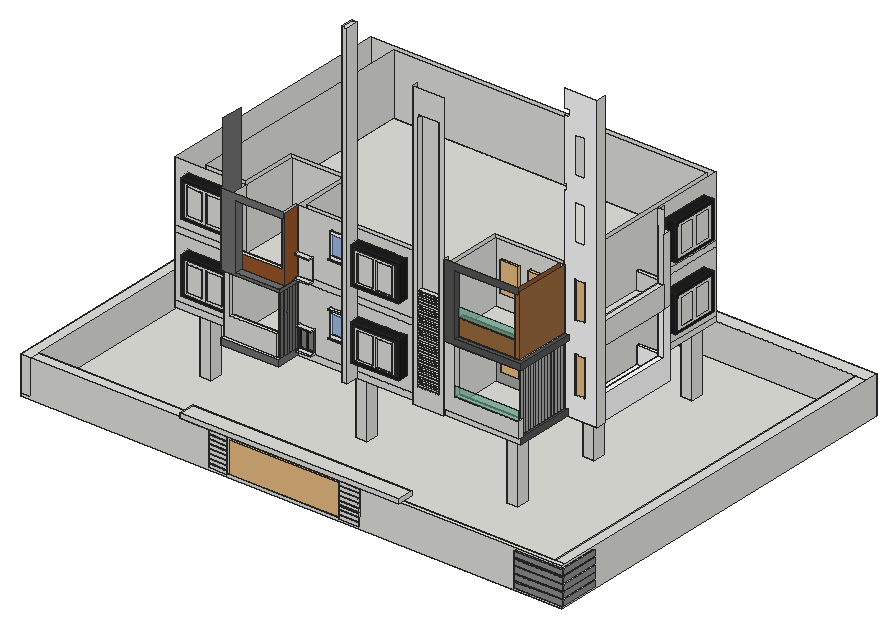
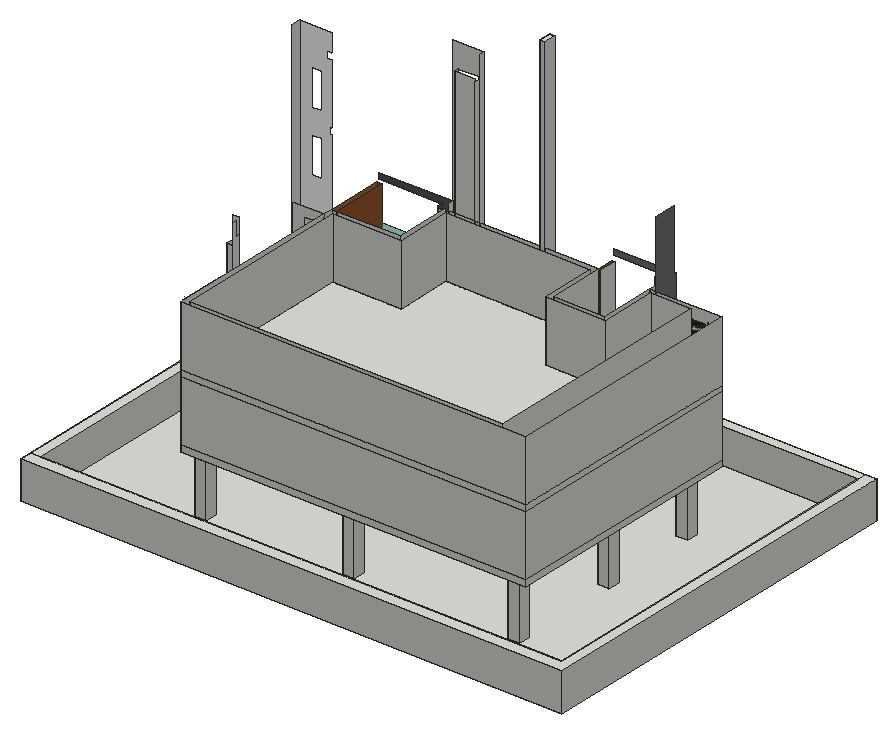
# SketchUp Ruby script. Lengths in inches.
U = 1.inch
M = Sketchup.active_model
def pt(a) = Geom::Point3d.new(a.map { |v| v * U })
def face(e, loops, mat)
  f = e.add_face(loops[0].map { |a| pt(a) })
  loops[1..].each { |l| e.add_face(l.map { |a| pt(a) }).erase! }
  f.material = f.back_material = mat if mat
  f
end
# faces: each face lists its corners as indices into pts; further lists are holes
def faces(e, pts, list, mat = nil) = list.each { |f| face(e, (f[0].is_a?(Array) ? f : [f]).map { |l| l.map { |i| pts[i] } }, mat) }
# xy, xz, yz: faces in a plane at the given z, y or x. An outline is a flat list of corners, or four numbers for a rectangle; further outlines are holes
def ring(l) = l.size == 4 ? [[l[0], l[1]], [l[2], l[1]], [l[2], l[3]], [l[0], l[3]]] : l.each_slice(2).to_a
def flat(e, list, mat, &to3) = list.each { |f| face(e, (f[0].is_a?(Array) ? f : [f]).map { |l| ring(l).map { |u, v| to3.(u, v) } }, mat) }
def xy(e, z, list, mat = nil) = flat(e, list, mat) { |x, y| [x, y, z] }
def xz(e, y, list, mat = nil) = flat(e, list, mat) { |x, z| [x, y, z] }
def yz(e, x, list, mat = nil) = flat(e, list, mat) { |y, z| [x, y, z] }
def lines(e, pts, list) = list.each { |a, b| e.add_line(pt(pts[a]), pt(pts[b])) }
# prism: a flat outline (further loops are holes) pulled along v
def prism(e, loops, v, mat = nil)
  f = face(e, loops, mat); d = Geom::Vector3d.new(v.map { |x| x * U })
  f.pushpull(f.normal.samedirection?(d) ? d.length : -d.length)
end
def box(e, o, s, mat = nil) = prism(e, [[o, [o[0] + s[0], o[1], o[2]], [o[0] + s[0], o[1] + s[1], o[2]], [o[0], o[1] + s[1], o[2]]]], [0, 0, s[2]], mat)
def at(x, y, z, deg = 0) = Geom::Transformation.translation(pt([x, y, z])) * Geom::Transformation.rotation(ORIGIN, Z_AXIS, deg.degrees)
def axes(o, x, y, z) = Geom::Transformation.new([*x, 0, *y, 0, *z, 0, *pt(o).to_a, 1])
def part(name) = M.definitions.add(name)
# library, detail: a bought-in or finely detailed component or shape, given as its bounding box
def library(name, o, s) = part(name).tap { |d| box(d.entities, o, s) }
def detail(e, o, s) = box(e.add_group.entities, o, s)
def put(e, d, t, mat = nil) = e.add_instance(d, t).tap { |i| i.material = mat if mat }
def group(e, t, mat = nil) = e.add_group.tap { |g| g.transformation = t; g.material = mat if mat }.entities
root = M.entities
M.materials.add("Glass_Tinted_Gray").color = [0, 0, 0]
M.materials["Glass_Tinted_Gray"].alpha = 0.125
M.materials.add("MaterialE").color = [182, 131, 172]
M.materials["MaterialE"].alpha = 0.66
M.materials.add("MaterialF").color = [114, 188, 161]
M.materials["MaterialF"].alpha = 0.66
M.materials.add("[0135_DarkGray]").color = [81, 81, 81]
M.materials.add("[Color M00]").color = [255, 255, 255]
M.materials.add("[Color M03]").color = [170, 170, 170]
M.materials.add("[Color M04]").color = [142, 142, 142]
M.materials.add("[Color M05]").color = [114, 114, 114]
M.materials.add("[Color M06]").color = [86, 86, 86]
M.materials.add("[Color M08]").color = [30, 30, 30]
M.materials.add("[Color_000]").color = [255, 255, 255]
M.materials.add("[Mirror 02]1").color = [229, 229, 229]
M.materials.add("[Terrazzo Light Blue]").color = [196, 214, 227]
M.materials.add("[Translucent Glass Blue]").color = [100, 149, 237]
M.materials["[Translucent Glass Blue]"].alpha = 0.5
M.materials.add("[Wood Cherry Original]").color = [152, 86, 42]
M.materials.add("[Wood Floor]").color = [155, 105, 61]
c1 = part("Group\#83")
box(c1.entities,[-12.25,0,-120],[22.4375,23.375,120])
c2 = library("Slatted gate assembly",[-0.09,68.76,-0.1],[160,5.32,60.06])
c3 = part("Group\#96")
box(c3.entities,[0,-1.1875,0],[36.6875,1.1875,6.49])
c4 = part("Group\#3")
box(c4.entities,[3,0,0],[2.8125,4.1875,120.875])
c5 = part("Group\#76")
box(c5.entities,[0,0,0],[4.8125,4.8125,120],"[Color M05]")
c6 = library("Single door",[0,0,0],[7.5,39.86,83.92])
c7 = part("Group\#75")
box(c7.entities,[0,-10.375,0],[28.375,10.375,2.5])
c8 = part("PENTEK_RP Fineline 50S_Sliding_DoorCase_E1")
box(c8.entities,[0,0,0],[1.51,3.66,99.27],"[0135_DarkGray]")
c9 = part("PENTEK_RP Fineline 50S_SlidingDooe_Case_E2")
box(c9.entities,[0,0,0],[96.25,3.66,1.51],"[0135_DarkGray]")
c10 = part("pentek_RP Fineline 50S_SlidingDoor_Case")
put(c10.entities,c8,at(97.76,0,0))
put(c10.entities,c9,at(1.51,0,0))
put(c10.entities,c8,at(0,0,0))
put(c10.entities,c9,at(1.51,0,97.76))
c11 = part("PENTEK_RP Fineline 50S_SlidingDoor_GlazingBead_2")
box(c11.entities,[0,0,0],[0.56,0.59,94.39],"[0135_DarkGray]")
c12 = part("PENTEK_RP Fineline 50S_SlidingDoor_Glass")
box(c12.entities,[0,0,0],[46.58,0.16,94.39],"Glass_Tinted_Gray")
c13 = part("PENTEK_RP Fineline 50S_SlidingDoor_GlazingBead")
box(c13.entities,[0,0,0],[45.47,0.59,0.56],"[0135_DarkGray]")
c14 = part("PENTEK_RP Fineline 50S_SlidingDoor_Leaf_E1")
xy(c14.entities,0,[[0,0,0.93,1.97],[0.93,1.57,1.49,1.97]],"[0135_DarkGray]")
xy(c14.entities,96.25,[[0,0,0.93,0,0.93,1.57,1.49,1.57,1.49,1.97,0,1.97]],"[0135_DarkGray]")
xz(c14.entities,0,[[0,0,0.93,96.25]],"[0135_DarkGray]")
xz(c14.entities,1.57,[[0.93,0,1.49,95.32],[0.93,95.32,1.49,96.25]],"[0135_DarkGray]")
xz(c14.entities,1.97,[[0,0,1.49,96.25]],"[0135_DarkGray]")
yz(c14.entities,0,[[0,0,1.97,96.25]],"[0135_DarkGray]")
yz(c14.entities,0.93,[[0,0,1.57,0.93],[0,0.93,1.57,95.32],[0,95.32,1.57,96.25]],"[0135_DarkGray]")
yz(c14.entities,1.49,[[1.57,0,1.97,95.32],[1.57,95.32,1.97,96.25]],"[0135_DarkGray]")
c15 = part("PENTEK_RP Fineline 50S_SlidingDoor_Leaf_E2")
xy(c15.entities,0,[[0,0,0,1.57,0.56,1.57,0.56,1.97,46.02,1.97,46.02,1.57,46.58,1.57,46.58,0]],"[0135_DarkGray]")
xy(c15.entities,0.93,[[0,0,46.58,1.57]],"[0135_DarkGray]")
xy(c15.entities,1.49,[[0.56,1.57,46.02,1.97]],"[0135_DarkGray]")
xz(c15.entities,0,[[0,0,46.58,0.93]],"[0135_DarkGray]")
xz(c15.entities,1.57,[[0,0,0.56,0.93],[46.02,0,46.58,0.93],[0.56,0.93,46.02,1.49]],"[0135_DarkGray]")
xz(c15.entities,1.97,[[0.56,0,46.02,1.49]],"[0135_DarkGray]")
yz(c15.entities,0,[[0,0,1.57,0.93]],"[0135_DarkGray]")
yz(c15.entities,0.56,[[1.57,0,1.97,0.93],[1.57,0.93,1.97,1.49]],"[0135_DarkGray]")
yz(c15.entities,46.02,[[1.57,0,1.97,0.93],[1.57,0.93,1.97,1.49]],"[0135_DarkGray]")
yz(c15.entities,46.58,[[0,0,1.57,0.93]],"[0135_DarkGray]")
c16 = part("PENTEK_RP Fineline S_SlidingDoor_Leaf1")
put(c16.entities,c11,at(0.93,0,0.93))
put(c16.entities,c11,at(46.96,0,0.93))
put(c16.entities,c12,at(1.49,1.42,0.93))
put(c16.entities,c13,at(1.49,0,0.93))
put(c16.entities,c12,at(1.49,0.59,0.93),"[Terrazzo Light Blue]")
put(c16.entities,c14,at(0,0,0))
put(c16.entities,c14,axes([48.44,0,0],[-1,0,0],[0,1,0],[0,0,1]))
put(c16.entities,c15,axes([0.93,0,96.25],[1,0,0],[0,1,0],[0,0,-1]))
put(c16.entities,c15,at(0.93,0,0))
put(c16.entities,c13,at(1.49,0,94.77))
c17 = part("PENTEK_RP Fineline 50S_SlidingDoor_Leaf2")
put(c17.entities,c12,at(1.49,1.42,0.93))
put(c17.entities,c13,at(1.49,0,94.77))
put(c17.entities,c11,at(46.96,0,0.93))
put(c17.entities,c12,at(1.49,0.59,0.93),"[Mirror 02]1")
put(c17.entities,c11,at(0.93,0,0.93))
put(c17.entities,c14,at(0,0,0))
put(c17.entities,c14,axes([48.44,0,0],[-1,0,0],[0,1,0],[0,0,1]))
put(c17.entities,c13,at(1.49,0,0.93))
put(c17.entities,c15,axes([0.93,0,96.25],[1,0,0],[0,1,0],[0,0,-1]))
put(c17.entities,c15,at(0.93,0,0))
c18 = part("PENTEK - Slimmest Steel Sliding Door / Window\#1")
put(c18.entities,c10,at(0,-1.88,-0.09))
put(c18.entities,c16,at(1.51,-2.27,1.42))
put(c18.entities,c17,at(49.32,-0.3,1.42))
c19 = library("Sliding Window",[0,0,0],[35.43,4.93,59.06])
c20 = part("Group\#4")
box(c20.entities,[0,0,0],[39.5625,8.625,2.78])
c21 = part("Window")
xy(c21.entities,31.72,[[-0.78,88.6,2.72,128.1]])
xy(c21.entities,34.95,[[-0.78,91.53,0.84,106.59],[0.84,91.53,1.05,97.58],[1.05,91.53,1.42,106.59],[1.42,91.53,2.72,106.59],[0.84,97.58,1.05,98.18],
  [0.84,98.18,1.05,106.59]])
xy(c21.entities,35.27,[[-0.78,110.09,0.97,125.14],[1.05,110.09,2.72,125.14]])
xy(c21.entities,58.35,[[2.72,108.74,3.8,109.74]])
xy(c21.entities,77.8125,[[-0.78,110.09,2.72,125.14],[0.97,110.09,1.05,125.14]])
xy(c21.entities,77.93,[[-0.78,91.53,0.84,106.59],[1.05,91.53,1.42,106.59],[1.42,91.53,2.72,106.59]])
xy(c21.entities,80.72,[[-0.78,88.6,2.72,128.1]])
xz(c21.entities,88.6,[[-0.78,31.72,2.72,80.72]])
xz(c21.entities,91.53,[[-0.78,34.95,0.84,77.93],[1.05,34.95,1.42,77.93],[1.42,34.95,2.72,77.93]])
xz(c21.entities,106.59,[[-0.78,34.95,0.84,77.93],[0.84,34.95,1.05,77.93],[0.84,34.95,2.72,77.93]])
xz(c21.entities,108.74,[[3.8,54.35,4.22,54.6,4.22,59.47,2.72,59.97,2.72,58.35,3.8,58.35]])
xz(c21.entities,109.74,[[3.8,54.35,3.8,58.35,2.72,58.35,2.72,59.97,4.22,59.47,4.22,54.6]])
xz(c21.entities,110.09,[[-0.78,35.27,0.97,77.8125],[1.05,35.27,2.72,77.8125]])
xz(c21.entities,125.14,[[-0.78,35.27,0.97,77.8125],[0.97,35.27,1.05,80.72],[1.05,35.27,2.72,77.8125]])
xz(c21.entities,128.1,[[-0.78,31.72,2.72,80.72]])
yz(c21.entities,-0.78,[[[88.6,31.72,128.1,80.72],[91.53,34.95,106.59,77.93],[110.09,35.27,125.14,77.8125]]])
yz(c21.entities,0.84,[[91.53,34.95,106.59,77.93]])
yz(c21.entities,0.97,[[110.09,35.27,125.14,77.8125]])
yz(c21.entities,1.05,[[91.53,34.95,106.59,77.93],[110.09,35.27,125.14,77.8125]])
yz(c21.entities,1.42,[[91.53,34.95,106.59,77.93]])
yz(c21.entities,2.72,[[[88.6,31.72,108.35,80.72],[91.53,34.95,106.59,77.93]],[[108.35,31.72,128.1,80.72],[110.09,35.27,125.14,77.8125],[108.74,58.35,109.74,59.97]]])
yz(c21.entities,3.8,[[108.74,54.35,109.74,58.35]])
yz(c21.entities,4.22,[[108.74,54.6,109.74,59.47]])
p = [[4.22,108.74,54.6],[3.8,108.74,54.35],[3.8,109.74,54.35],[4.22,109.74,54.6],[2.72,109.74,59.97],[2.72,108.74,59.97],
  [4.22,108.74,59.47],[4.22,109.74,59.47],[-0.78,86.4,89.94],[-0.78,86.44,89.94],[15.22,130.69,89.94],[15.22,130.65,89.94],
  [-0.78,86.44,28.19],[-0.78,86.4,28.19],[7.72,130.69,89.94],[7.72,130.65,89.94]]
faces(c21.entities,p,[[0,1,2,3],[4,5,6,7]])
lines(c21.entities,p,[[8,9],[10,11],[12,13],[14,15]])
c22 = part("Group\#5")
xy(c22.entities,0,[[[0,0,93.5,72.0625],[5.4,5.4,88.1,66.66]],[5.4,5.4,88.1,66.66]])
xy(c22.entities,20.1875,[[[0,0,93.5,72.0625],[5.4,5.4,88.1,66.66]]])
xz(c22.entities,0,[[0,0,93.5,20.1875]])
xz(c22.entities,5.4,[[5.4,0,88.1,20.1875]])
xz(c22.entities,66.66,[[5.4,0,88.1,20.1875]])
xz(c22.entities,72.0625,[[0,0,93.5,20.1875]])
yz(c22.entities,0,[[0,0,72.0625,20.1875]])
yz(c22.entities,5.4,[[5.4,0,66.66,20.1875]])
yz(c22.entities,88.1,[[5.4,0,66.66,20.1875]])
yz(c22.entities,93.5,[[0,0,72.0625,20.1875]])
c23 = part("glassE")
xy(c23.entities,0,[[0,0,37.99,0.79]],"MaterialE")
xy(c23.entities,38.27,[[0,0,37.99,0.79]],"MaterialE")
xz(c23.entities,0,[[0,0,37.99,38.27]],"MaterialF")
yz(c23.entities,0,[[0,0,0.79,38.27]],"MaterialE")
yz(c23.entities,37.99,[[0,0,0.79,38.27]],"MaterialE")
c24 = library("grille P1",[0,0,0],[0.79,28.9,72.83])
c25 = part("Group\#73")
box(c25.entities,[0,0,0],[34.1875,2.25,6.125])
c26 = part("bod vindu")
g1 = group(c26.entities,at(0,-46.85,0),"[Translucent Glass Blue]")
yz(g1,0.94,[[2.36,2.36,44.49,19.65]],"[Translucent Glass Blue]")
p = [[0.55,44.49,2.36],[0.94,44.49,2.36],[0.55,2.36,19.65],[0.94,2.36,19.65]]
lines(g1,p,[[0,1],[2,3]])
g2 = group(g1,at(0,46.85,0,-90),"[Color_000]")
xy(g2,0,[[0,0,46.85,3.9375]])
xy(g2,1.57,[[1.57,0,45.28,0.55]])
xy(g2,2.36,[[2.36,0.55,44.49,3.9375]])
xy(g2,19.65,[[2.36,0.55,4.29,3.9375],[4.29,0.55,44.49,3.9375]])
xy(g2,20.43,[[1.57,0,45.28,0.55]])
xy(g2,22.01,[[0,0,46.85,3.9375]])
xz(g2,0,[[[0,0,46.85,22.01],[1.57,1.57,45.28,20.43]]])
xz(g2,0.55,[[1.57,1.57,45.28,2.36],[1.57,2.36,2.36,2.36,2.36,19.65,44.49,19.65,44.49,2.36,45.28,2.36,45.28,20.43,1.57,20.43]])
xz(g2,3.9375,[[[0,0,46.85,22.01],[2.36,2.36,44.49,19.65]]])
yz(g2,0,[[0,0,3.9375,22.01]])
yz(g2,1.57,[[0,1.57,0.55,2.36,0.55,20.43,0,20.43]])
yz(g2,2.36,[[0.55,2.36,3.9375,19.65]])
yz(g2,44.49,[[0.55,2.36,3.9375,19.65]])
yz(g2,45.28,[[0,1.57,0,20.43,0.55,20.43,0.55,2.36]])
yz(g2,46.85,[[0,0,3.9375,22.01]])
p = [[45.28,0,1.57],[1.57,0,1.57],[1.57,0.55,2.36],[2.36,0.55,2.36],[44.49,0.55,2.36],[45.28,0.55,2.36]]
faces(g2,p,[[0,1,2,3,4,5]])
xy(root,-137.6875,[[0,11.875,1063.6875,784.3125]])
xy(root,-132,[[407.01,11.875,626.4,11.875,626.4,20.5625,1043.76,20.5625,1043.76,759.59,20.58,759.59,20.58,31.625,407.01,31.625]])
xy(root,-131.51,[[1063.6875,11.875,1067.5625,87.875]])
xy(root,-120.77,[[1063.6875,11.875,1067.5625,87.875]])
xy(root,-118.08,[[1063.6875,11.875,1067.5625,87.875]])
xy(root,-107.34,[[1063.6875,11.875,1067.5625,87.875]])
xy(root,-104.92,[[1063.6875,11.875,1067.5625,87.875]])
xy(root,-94.18,[[1063.6875,11.875,1067.5625,87.875]])
xy(root,-91.42,[[1063.6875,11.875,1067.5625,87.875]])
xy(root,-80.68,[[1063.6875,11.875,1067.5625,87.875]])
xy(root,-76.99,[[1063.6875,11.875,1067.5625,87.875]])
xy(root,-66.25,[[1063.6875,11.875,1067.5625,87.875]])
xy(root,-63.1875,[[0,11.875,20.58,11.875,20.58,759.59,1063.6875,759.59,1063.6875,784.3125,0,784.3125],[20.58,11.875,370.32,31.625],[667.3,11.875,1063.6875,20.5625],[1043.76,20.5625,1063.6875,759.59]])
xy(root,-57.5,[[322.88,0,322.88,31.625,370.32,31.625,370.32,11.875,349.63,11.875,349.63,0],[349.63,0,407.01,11.875],[407.01,0,407.01,31.625,626.4,31.625,626.4,11.875,688.36,11.875,688.36,0],[742.8,0,742.8,11.875,667.3,11.875,667.3,31.625,752.38,31.625,752.38,0],[688.36,0,742.8,11.875],
  [626.4,11.875,667.3,20.5625],[626.4,20.5625,667.3,31.625]])
xy(root,-49,[[322.88,0,752.38,31.625]])
xy(root,-12,[[278.57,155.5,392.02,203.9375],[685.61,198,685.61,203.9375,827.97,203.9375,827.97,313.75,833.78,313.75,833.78,198],[827.97,313.75,891.78,332.62]])
xy(root,-12,[[624.38,194.4375,685.61,203.9375],[827.97,332.62,887.97,496.51]],"[Color M00]")
xy(root,0,[[278.57,155.5,392.02,162.81],[383.02,162.81,392.02,169.625],[291.32,169.625,392.02,313.75],[685.61,194.4375,833.78,198],[685.61,198,833.78,203.9375],
  [[150.47,203.9375,291.32,203.9375,291.32,313.75,392.02,313.75,392.02,203.9375,693.39,203.9375,693.39,313.75,827.97,313.75,827.97,683.9375,150.47,683.9375],[203.47,212.9375,203.47,674.9375,818.97,674.9375,818.97,322.75,684.39,322.75,684.39,212.9375,401.02,212.9375,401.02,322.75,282.32,322.75,282.32,212.9375]],[693.39,203.9375,827.97,313.75],[203.47,212.9375,282.32,212.9375,282.32,322.75,401.02,322.75,401.02,212.9375,684.39,212.9375,684.39,322.75,818.97,322.75,818.97,674.9375,203.47,674.9375]])
xy(root,0,[[827.97,332.62,876.25,489.82]],"[Color M00]")
xy(root,0,[[827.97,203.9375,833.78,313.75]],"[Color M06]")
xy(root,22.35,[[635.73,194.4375,675.23,203.0625]])
xy(root,30.3125,[[707.95,194.4375,833.78,203.9375]])
xy(root,30.85,[[848.78,313.75,867.09,332.62]])
xy(root,33.25,[[827.97,489.82,876.25,496.51]],"[Color M00]")
xy(root,35.3125,[[876.25,332.62,887.97,481.58]],"[Color M00]")
xy(root,40.0625,[[291.32,162.81,383.02,169.625]])
xy(root,101.98,[[848.78,313.75,867.09,332.62]])
xy(root,120,[[685.61,194.4375,707.95,203.9375],[707.95,194.4375,707.95,203.9375,827.97,203.9375,827.97,313.75,836.28,313.75,836.28,194.4375],[[150.47,203.9375,291.32,203.9375,291.32,313.75,392.02,313.75,392.02,203.9375,693.39,203.9375,693.39,313.75,827.97,313.75,827.97,683.9375,150.47,683.9375],[203.47,212.9375,203.47,674.9375,818.97,674.9375,818.97,322.75,684.39,322.75,684.39,212.9375,401.02,212.9375,401.02,322.75,282.32,322.75,282.32,212.9375]],[827.97,332.62,887.97,496.51]])
xy(root,120,[[278.57,155.5,278.57,162.81,291.32,162.81,291.32,203.9375,395.4,203.9375,395.4,155.5]],"[Color M05]")
xy(root,125.21,[[308.96,155.5,392.02,170.3125],[392.02,155.5,395.4,203.9375]],"[Color M05]")
xy(root,128.18,[[392.46,203.9375,420.84,205.375]])
xy(root,132,[[[150.47,203.9375,291.32,203.9375,291.32,313.75,392.02,313.75,392.02,203.9375,392.46,203.9375,392.46,205.5,420.84,205.5,420.84,203.9375,693.39,203.9375,693.39,313.75,827.97,313.75,827.97,683.9375,150.47,683.9375],[203.47,212.9375,203.47,674.9375,818.97,674.9375,818.97,322.75,684.39,322.75,684.39,212.9375,401.02,212.9375,401.02,322.75,282.32,322.75,282.32,212.9375]],[291.32,203.9375,392.02,313.75],[693.39,203.9375,708.18,203.9375,708.18,214.1875,816.45,214.1875,816.45,313.75,693.39,313.75],[708.18,203.9375,816.45,214.1875],[816.45,203.9375,818.5,214.1875],
  [818.5,203.9375,827.97,313.75],[392.46,205.375,420.84,205.5],[203.47,212.9375,282.32,212.9375,282.32,322.75,401.02,322.75,401.02,212.9375,684.39,212.9375,684.39,322.75,818.97,322.75,818.97,674.9375,203.47,674.9375],[816.45,214.1875,818.5,313.75],[827.97,332.62,876.25,488.11]])
xy(root,132,[[707.95,194.4375,836.28,194.4375,836.28,313.75,827.97,313.75,827.97,203.9375,707.95,203.9375]],"[Color M06]")
xy(root,132.08,[[291.14,177.25,386.69,203.9375]])
xy(root,152.52,[[291.14,170.3125,386.69,177.25]])
xy(root,162.85,[[848.78,313.75,867.09,332.62]])
xy(root,163.05,[[876.25,332.62,887.97,481.58]])
xy(root,163.875,[[827.97,488.11,876.25,496.51]])
xy(root,165.1875,[[708.18,203.9375,818.5,214.1875]],"[Wood Cherry Original]")
xy(root,168.56,[[392.46,203.9375,420.84,205.375],[392.46,205.375,420.84,205.5]])
xz(root,0,[[322.88,-57.5,752.38,-49]])
xz(root,11.875,[[0,-137.6875,1063.6875,-137.6875,1063.6875,-63.1875,1047.02,-63.1875,1047.02,-76.99,972.52,-76.99,972.52,-63.1875,667.3,-63.1875,667.3,-57.5,626.4,-57.5,626.4,-132,407.01,-132,407.01,-63.99,370.32,-63.99,370.32,-63.1875,20.58,-63.1875,20.58,-132,0,-132],[0,-132,20.58,-63.1875],[1063.6875,-131.51,1067.5625,-120.77],[1063.6875,-118.08,1067.5625,-107.34],[1063.6875,-104.92,1067.5625,-94.18],
  [1063.6875,-91.42,1067.5625,-80.68],[1063.6875,-76.99,1067.5625,-66.25],[972.52,-66.25,1047.02,-63.1875]])
xz(root,20.5625,[[626.4,-132,626.4,-57.5,667.3,-57.5,667.3,-63.1875,1043.76,-63.1875,1043.76,-132]])
xz(root,31.625,[[20.58,-132,20.58,-63.1875,370.32,-63.1875,370.32,-57.5,322.88,-57.5,322.88,-49,752.38,-49,752.38,-57.5,407.01,-57.5,407.01,-132]])
xz(root,87.875,[[1063.6875,-131.51,1067.5625,-120.77],[1063.6875,-118.08,1067.5625,-107.34],[1063.6875,-104.92,1067.5625,-94.18],[1063.6875,-91.42,1067.5625,-80.68],[1063.6875,-76.99,1067.5625,-66.25]])
xz(root,155.5,[[278.57,-12,392.02,0],[278.57,120,395.4,120,395.4,125.21,308.96,125.21,308.96,252,400.83,252,400.83,264,278.57,264]],"[Color M05]")
xz(root,162.81,[[278.57,0,383.02,0,383.02,40.0625,291.32,40.0625,291.32,120,278.57,120]])
xz(root,169.625,[[291.32,0,383.02,40.0625]])
xz(root,170.3125,[[291.14,152.52,308.96,252]])
xz(root,170.3125,[[308.96,125.21,392.02,125.21,392.02,252,386.69,252,386.69,152.52,308.96,152.52]],"[Wood Cherry Original]")
xz(root,177.25,[[291.14,132.08,386.69,152.52]])
xz(root,194.4375,[[[624.38,-12,685.61,548.1875],[635.73,22.35,675.23,501.53]],[685.61,0,833.78,0,833.78,30.3125,707.95,30.3125,707.95,120,685.61,120]])
xz(root,194.4375,[[685.61,120,836.28,120,836.28,132,707.95,132,707.95,252.02,830.59,252.02,830.59,264,685.61,264]],"[Color M06]")
xz(root,198,[[685.61,-12,833.78,0]])
xz(root,203.0625,[[635.73,22.35,675.23,501.53]])
xz(root,203.9375,[[624.38,-12,685.61,0],[685.61,-12,827.97,0],[150.47,0,278.57,120],[392.02,0,624.38,120],[624.38,0,685.61,120],
  [685.61,0,693.39,120],[693.39,0,693.39,19.1875,707.95,19.1875,707.95,30.3125,833.78,30.3125,833.78,0],[693.39,19.1875,707.95,120],[150.47,120,278.57,132],[278.57,120,278.57,132,392.02,132,392.02,125.21,395.4,125.21,395.4,120],
  [395.4,120,624.38,120,624.38,132,420.84,132,420.84,128.18,392.46,128.18,392.46,132,392.02,132,392.02,125.21,395.4,125.21],[624.38,120,685.61,132],[685.61,120,827.97,132],[392.46,128.18,420.84,168.56],[150.47,132,278.57,252],
  [278.57,132,291.32,132,291.32,132.08,291.14,132.08,291.14,252,278.57,252],[291.32,132,291.32,132.08,386.69,132.08,386.69,252,392.02,252,392.02,132],[392.02,132,392.46,132,392.46,168.56,420.84,168.56,420.84,132,497.83,132,497.83,252,392.02,252],[508.2,132,624.38,252],[624.38,132,685.61,252],
  [685.61,132,693.39,249.15],[693.39,132,707.95,249.15],[291.14,132.08,291.32,252]])
xz(root,203.9375,[[708.18,132,818.5,165.1875],[818.5,132,827.97,252]],"[Wood Floor]")
xz(root,205.375,[[392.46,132,420.84,168.56]])
xz(root,205.5,[[392.46,132,420.84,168.56]])
xz(root,212.9375,[[203.47,0,282.32,120],[401.02,0,684.39,120],[203.47,132,282.32,252],[401.02,132,684.39,252]])
xz(root,214.1875,[[708.18,132,818.5,165.1875]])
xz(root,313.75,[[291.32,0,392.02,120],[291.32,132,392.02,252],[693.39,132,818.5,252],[818.5,132,827.97,252]])
xz(root,313.75,[[827.97,-12,832.47,0],[[833.78,-12,891.78,-12,891.78,562.75,827.97,562.75,827.97,528,838.2,528,838.2,516,827.97,516,827.97,396,832.47,396,832.47,384,827.97,384,827.97,132,836.28,132,836.28,120,827.97,120,827.97,0,833.78,0],[848.78,30.85,867.09,101.98],[848.78,162.85,867.09,233.98],[848.78,298.79,867.09,369.91],[848.78,417.54,867.09,488.67],[828.01,252,830.59,264]],[832.47,-12,833.78,0]],"[Color M00]")
xz(root,313.75,[[693.39,0,827.97,120]],"[Color M03]")
xz(root,313.75,[[827.97,120,832.47,132],[832.47,120,836.28,132]],"[Color M06]")
xz(root,322.75,[[282.32,0,401.02,120],[684.39,0,818.97,120],[282.32,132,401.02,252],[684.39,132,818.97,252]])
xz(root,332.62,[[827.97,-12,827.97,0,876.25,0,876.25,35.3125,887.97,35.3125,887.97,-12],[887.97,-12,891.78,35.3125],[[827.97,0,827.97,120,891.78,120,891.78,35.3125,876.25,35.3125,876.25,0],[848.78,30.85,867.09,101.98]],[827.97,120,827.97,132,876.25,132,876.25,163.05,887.97,163.05,887.97,120],[887.97,120,891.78,163.05],
  [[827.97,132,827.97,252,891.78,252,891.78,163.05,876.25,163.05,876.25,132],[848.78,162.85,867.09,233.98]]])
xz(root,481.58,[[876.25,163.05,887.97,163.05,887.97,295.27,877.14,295.27,877.14,264,876.25,264]])
xz(root,481.58,[[876.25,35.3125,887.97,163.05]],"[Color M00]")
xz(root,488.11,[[827.97,132,876.25,163.875]])
xz(root,489.82,[[827.97,0,876.25,33.25]],"[Color M00]")
xz(root,496.51,[[827.97,120,876.25,163.875],[876.25,120,887.97,252]])
xz(root,496.51,[[827.97,-12,887.97,-12,887.97,120,876.25,120,876.25,33.25,827.97,33.25]],"[Color M00]")
xz(root,674.9375,[[203.47,0,818.97,120],[203.47,132,818.97,252]])
xz(root,683.9375,[[150.47,0,827.97,120],[150.47,120,827.97,132],[150.47,132,827.97,252]])
xz(root,759.59,[[20.58,-132,1043.76,-63.1875]])
xz(root,784.3125,[[0,-137.6875,1063.6875,-63.1875]])
yz(root,0,[[11.875,-137.6875,784.3125,-63.1875]])
yz(root,20.58,[[31.625,-132,759.59,-63.1875]])
yz(root,150.47,[[203.9375,0,683.9375,120],[203.9375,120,683.9375,132],[203.9375,132,683.9375,252]])
yz(root,203.47,[[212.9375,0,674.9375,120],[212.9375,132,674.9375,252]])
yz(root,278.57,[[162.81,0,203.9375,120]])
yz(root,278.57,[[155.5,-12,203.9375,0],[155.5,120,155.5,264,160.4375,264,160.4375,384,203.9375,384,203.9375,120]],"[Color M05]")
yz(root,282.32,[[212.9375,0,322.75,120],[212.9375,132,322.75,252]])
yz(root,291.14,[[177.25,132.08,203.9375,132.08,203.9375,252,170.3125,252,170.3125,152.52,177.25,152.52]])
yz(root,291.32,[[169.625,0,313.75,120],[162.81,40.0625,169.625,120],[203.9375,132,313.75,252]])
yz(root,308.96,[[155.5,125.21,170.3125,252]],"[Color M05]")
yz(root,322.88,[[0,-57.5,31.625,-49]])
yz(root,370.32,[[11.875,-63.1875,31.625,-57.5]])
yz(root,383.02,[[162.81,0,169.625,40.0625]])
yz(root,386.69,[[177.25,132.08,177.25,152.52,170.3125,152.52,170.3125,252,203.9375,252,203.9375,132.08]])
yz(root,392.02,[[203.9375,0,313.75,120],[203.9375,132,313.75,252]])
yz(root,392.02,[[155.5,-12,203.9375,0]],"[Color M05]")
yz(root,392.02,[[170.3125,125.21,203.9375,252]],"[Wood Cherry Original]")
yz(root,392.46,[[203.9375,128.18,205.375,132],[203.9375,132,205.375,168.56],[205.375,132,205.5,168.56]])
yz(root,395.4,[[155.5,120,203.9375,125.21]],"[Color M05]")
yz(root,401.02,[[212.9375,0,322.75,120],[212.9375,132,322.75,252]])
yz(root,407.01,[[11.875,-132,31.625,-57.5]])
yz(root,420.84,[[203.9375,128.18,205.375,132],[203.9375,132,205.375,168.56],[205.375,132,205.5,168.56]])
yz(root,624.38,[[194.4375,-12,203.9375,548.1875]])
yz(root,626.4,[[11.875,-132,20.5625,-57.5]])
yz(root,635.73,[[194.4375,22.35,203.0625,494.88]])
yz(root,667.3,[[11.875,-63.1875,20.5625,-57.5]])
yz(root,675.23,[[194.4375,22.35,203.0625,501.53]])
yz(root,684.39,[[212.9375,0,322.75,120],[212.9375,132,322.75,252]])
yz(root,685.61,[[198,-12,203.9375,0],[194.4375,0,203.9375,120],[194.4375,120,203.9375,264]])
yz(root,685.61,[[194.4375,-12,198,0]],"[Color M00]")
yz(root,693.39,[[203.9375,0,313.75,120],[203.9375,132,313.75,252]])
yz(root,707.95,[[194.4375,30.3125,203.9375,120]])
yz(root,707.95,[[194.4375,132,203.9375,252.02]],"[Color M06]")
yz(root,708.18,[[203.9375,132,214.1875,165.1875]])
yz(root,752.38,[[0,-57.5,31.625,-49]])
yz(root,818.5,[[203.9375,132,214.1875,165.1875]])
yz(root,818.5,[[214.1875,132,214.1875,165.1875,203.9375,165.1875,203.9375,252,313.75,252,313.75,132]],"[Wood Cherry Original]")
yz(root,818.97,[[322.75,0,674.9375,120],[322.75,132,674.9375,252]])
yz(root,827.97,[[313.75,-12,332.62,0],[313.75,0,332.62,120],[332.62,0,489.82,0,489.82,33.25,496.51,33.25,496.51,0,683.9375,0,683.9375,120,332.62,120],[203.9375,120,313.75,132],[313.75,120,332.62,132],
  [496.51,120,683.9375,132],[313.75,132,332.62,252],[332.62,132,488.11,132,488.11,163.875,496.51,163.875,496.51,132,683.9375,132,683.9375,252,332.62,252],[488.11,132,496.51,163.875]])
yz(root,827.97,[[203.9375,-12,313.75,0],[489.82,0,496.51,33.25]],"[Color M00]")
yz(root,827.97,[[203.9375,132,313.75,252]],"[Wood Floor]")
yz(root,833.78,[[194.4375,0,203.9375,30.3125]])
yz(root,833.78,[[198,-12,313.75,0]],"[Color M06]")
yz(root,836.28,[[194.4375,120,313.75,132]],"[Color M06]")
yz(root,848.78,[[313.75,30.85,332.62,101.98],[313.75,162.85,332.62,233.98]])
yz(root,867.09,[[313.75,30.85,332.62,101.98],[313.75,162.85,332.62,233.98]])
yz(root,876.25,[[332.62,132,481.58,163.05],[481.58,132,481.58,264,490.24,264,490.24,292.1875,496.51,292.1875,496.51,163.875,488.11,163.875,488.11,132]])
yz(root,876.25,[[332.62,0,489.82,0,489.82,33.25,496.51,33.25,496.51,163.875,488.11,163.875,488.11,132,481.58,132,481.58,35.3125,332.62,35.3125]],"[Color M00]")
yz(root,887.97,[[332.62,120,481.58,163.05],[481.58,120,496.51,252]])
yz(root,887.97,[[332.62,-12,332.62,35.3125,481.58,35.3125,481.58,120,496.51,120,496.51,-12]],"[Color M00]")
yz(root,891.78,[[313.75,-12,332.62,562.75]])
yz(root,1043.76,[[20.5625,-132,759.59,-63.1875]])
yz(root,1063.6875,[[11.875,-137.6875,784.3125,-137.6875,784.3125,-63.1875,11.875,-63.1875,11.875,-66.25,87.875,-66.25,87.875,-76.99,11.875,-76.99,11.875,-80.68,87.875,-80.68,87.875,-91.42,11.875,-91.42,11.875,-94.18,87.875,-94.18,87.875,-104.92,11.875,-104.92,11.875,-107.34,87.875,-107.34,87.875,-118.08,11.875,-118.08,11.875,-120.77,87.875,-120.77,87.875,-131.51,11.875,-131.51],[11.875,-131.51,87.875,-120.77],[11.875,-118.08,87.875,-107.34],[11.875,-104.92,87.875,-94.18],[11.875,-91.42,87.875,-80.68],
  [11.875,-76.99,87.875,-66.25]])
yz(root,1067.5625,[[11.875,-131.51,87.875,-120.77],[11.875,-118.08,87.875,-107.34],[11.875,-104.92,87.875,-94.18],[11.875,-91.42,87.875,-80.68],[11.875,-76.99,87.875,-66.25]],"[Color M04]")
g3 = group(root,at(626.4,11.875,-132.91))
box(g3,[0,-1.1875,0],[38.5625,1.1875,6.49])
put(root,c1,at(809.27,210.35,-12))
put(root,c1,at(809.27,396.91,-12))
put(root,c1,at(809.27,637.53,-12))
put(root,c1,at(193.77,637.53,-12))
put(root,c1,at(518.65,637.53,-12))
put(root,c1,at(193.77,417.41,-12))
put(root,c1,at(193.77,224.85,-12))
put(root,c1,at(500.65,224.85,-12))
put(root,c2,axes([407.13,-54.76,-131.9],[1.38923,0,0],[0,1,0],[0,0,1]))
put(root,c3,at(370.32,11.875,-131.99))
g4 = group(root,at(972.52,11.875,-131.51),"[Color M04]")
box(g4,[0,-2.875,0],[95.04,2.875,10.74])
g5 = group(root,at(626.4,11.875,-124.41))
box(g5,[0,-1.1875,0],[38.5625,1.1875,6.49])
put(root,c3,at(370.32,11.875,-123.49))
g6 = group(root,at(972.52,11.875,-118.08),"[Color M04]")
box(g6,[0,-2.875,0],[95.04,2.875,10.74])
g7 = group(root,at(626.4,11.875,-115.91))
box(g7,[0,-1.1875,0],[39.875,1.1875,6.49])
put(root,c3,at(370.32,11.875,-114.99))
g8 = group(root,at(626.4,11.875,-107.41))
box(g8,[0,-1.1875,0],[39.875,1.1875,6.49])
put(root,c3,at(370.32,11.875,-106.49))
g9 = group(root,at(972.52,11.875,-104.92),"[Color M04]")
box(g9,[0,-2.875,0],[95.04,2.875,10.74])
g10 = group(root,at(626.4,11.875,-98.91))
box(g10,[0,-1.1875,0],[40.9,1.1875,6.49])
put(root,c3,at(370.32,11.875,-97.99))
g11 = group(root,at(972.52,11.875,-91.42),"[Color M04]")
box(g11,[0,-2.875,0],[95.04,2.875,10.74])
g12 = group(root,at(626.4,11.875,-90.41))
box(g12,[0,-1.1875,0],[40.9,1.1875,6.49])
put(root,c3,at(370.32,11.875,-89.49))
g13 = group(root,at(626.4,11.875,-81.91))
box(g13,[0,-1.1875,0],[40.9,1.1875,6.49])
put(root,c3,at(370.32,11.875,-80.99))
g14 = group(root,at(972.52,11.875,-76.99),"[Color M04]")
box(g14,[0,-2.875,0],[95.04,2.875,10.74])
g15 = group(root,at(626.4,11.875,-73.41))
box(g15,[0,-1.1875,0],[40.9,1.1875,6.49])
put(root,c3,at(370.32,11.875,-72.49))
g16 = group(root,at(626.4,11.875,-64.91))
box(g16,[0,-1.1875,0],[40.9,1.1875,6.49])
put(root,c3,at(370.32,11.875,-63.99))
g17 = group(root,at(193.09,683.9375,-12))
box(g17,[-42.625,-480,0],[677.5,480,12])
g18 = group(root,at(497.83,203.9375,132))
box(g18,[0,-24.3125,-144],[10.37,24.3125,626.4375])
put(root,c4,at(822.16,206.24,0),"[Color M03]")
put(root,c4,at(822.16,212.62,0),"[Color M03]")
put(root,c4,at(822.16,218.68,0),"[Color M03]")
put(root,c4,at(822.16,224.93,0),"[Color M03]")
put(root,c4,at(822.16,230.87,0),"[Color M03]")
put(root,c4,at(822.16,237.31,0),"[Color M03]")
put(root,c4,at(822.16,243.62,0),"[Color M03]")
put(root,c4,at(822.16,250.43,0),"[Color M03]")
put(root,c4,at(822.16,257.9,0),"[Color M03]")
put(root,c4,at(822.16,265.15,0),"[Color M03]")
put(root,c4,at(822.16,273.03,0),"[Color M03]")
put(root,c4,at(822.16,280.9,0),"[Color M03]")
put(root,c4,at(822.16,289.46,0),"[Color M03]")
put(root,c4,at(822.16,296.96,0),"[Color M03]")
put(root,c4,at(822.16,304.71,0),"[Color M03]")
put(root,c5,at(385.41,201.05,0))
put(root,c5,at(385.41,193.73,0))
put(root,c5,at(385.41,186.36,0))
put(root,c5,at(385.41,179.55,0))
put(root,c5,at(385.41,172.8,0))
put(root,c5,at(385.41,164.89,0))
put(root,c6,at(760.44,316.08,0,-90))
put(root,c7,at(396.15,203.9375,0.24))
put(root,c18,axes([396.44,203.15,3.43],[0.27919,0,0],[0,0.34311,0],[0,0,0.40008]))
put(root,c19,at(705.78,308.67,22.64))
put(root,c20,at(635.73,194.4375,24.13))
put(root,c21,axes([778.5,184.53,-8.6],[0,1,0],[-2.03871,0,0],[0,0,1.22883]))
put(root,c21,axes([444.25,184.53,-8.6],[0,1,0],[-2.03871,0,0],[0,0,1.22883]))
put(root,c22,axes([512.06,203.9375,26.04],[1,0,0],[0,0,1],[0,-1,0]),"[Color M08]")
put(root,c22,axes([177.81,203.9375,26.04],[1,0,0],[0,0,1],[0,-1,0]),"[Color M08]")
put(root,c20,at(635.73,194.4375,29.88))
put(root,c23,axes([707.95,194.3,30.3125],[3.31,0,0],[0,1.17,0],[0,0,0.5016]))
put(root,c24,axes([867.09,313.75,30.47],[0,1,0],[-0.61577,0,0],[0,0,0.98]))
put(root,c21,axes([852.91,821.1,-2.91],[-1,0,0],[0,-2.03871,0],[0,0,1.22883]))
put(root,c22,axes([833.5,554.66,31.73],[0,1,0],[0,0,1],[1,0,0]),"[Color M08]")
put(root,c20,at(635.73,194.4375,35.63))
put(root,c20,at(635.73,194.4375,41.38))
put(root,c25,axes([456.17,203.9375,41.61],[1,0,0],[0,0,1],[0,-1,0]))
put(root,c7,at(396.15,203.9375,43.11))
put(root,c26,axes([488.85,203.9375,43.86],[0,-1,0],[0.6656,0,0],[0,0,2.2308]))
put(root,c20,at(635.73,194.4375,47.13))
put(root,c20,at(635.73,194.4375,52.88))
put(root,c20,at(635.73,194.4375,58.63))
put(root,c20,at(635.73,194.4375,64.38))
put(root,c20,at(635.73,194.4375,70.13))
put(root,c20,at(635.73,194.4375,75.88))
put(root,c20,at(635.73,194.4375,81.63))
put(root,c20,at(635.73,194.4375,87.38))
put(root,c25,axes([456.17,203.9375,92.96],[1,0,0],[0,0,1],[0,-1,0]))
put(root,c20,at(635.73,194.4375,93.13))
put(root,c20,at(635.73,194.4375,98.88))
put(root,c20,at(635.73,194.4375,104.63))
put(root,c20,at(635.73,194.4375,110.38))
put(root,c20,at(635.73,194.4375,116.13))
put(root,c20,at(635.73,194.4375,121.88))
put(root,c7,at(392.46,203.9375,125.68))
put(root,c20,at(635.73,194.4375,127.63))
put(root,c20,at(635.73,194.4375,133.38))
put(root,c6,at(760.44,316.08,136.5,-90))
put(root,c20,at(635.73,194.4375,139.13))
put(root,c20,at(635.73,194.4375,144.88))
put(root,c20,at(635.73,194.4375,150.63))
put(root,c20,at(635.73,194.4375,156.38))
put(root,c21,axes([852.91,821.1,124.09],[-1,0,0],[0,-2.03871,0],[0,0,1.22883]))
put(root,c22,axes([833.5,554.66,158.73],[0,1,0],[0,0,1],[1,0,0]),"[Color M08]")
put(root,c19,at(704.35,308.67,160.625))
put(root,c21,axes([778.5,184.53,126.96],[0,1,0],[-2.03871,0,0],[0,0,1.22883]))
put(root,c21,axes([444.25,184.53,126.96],[0,1,0],[-2.03871,0,0],[0,0,1.22883]))
put(root,c22,axes([512.06,203.9375,161.6],[1,0,0],[0,0,1],[0,-1,0]),"[Color M08]")
put(root,c22,axes([177.81,203.9375,161.6],[1,0,0],[0,0,1],[0,-1,0]),"[Color M08]")
put(root,c20,at(635.73,194.4375,162.13))
put(root,c24,axes([867.09,313.75,162.6],[0,1,0],[-0.61577,0,0],[0,0,0.98]))
put(root,c23,axes([708.18,203.9375,165.1875],[2.9128,0,0],[0,1.17,0],[0,0,0.5016]))
put(root,c20,at(635.73,194.4375,167.88))
put(root,c7,at(392.46,203.9375,168.56))
put(root,c20,at(635.73,194.4375,173.63))
put(root,c20,at(635.73,194.4375,179.2))
put(root,c25,axes([456.17,203.9375,179.99],[1,0,0],[0,0,1],[0,-1,0]))
put(root,c26,axes([488.85,203.9375,182.24],[0,-1,0],[0.6656,0,0],[0,0,2.2308]))
put(root,c20,at(635.73,194.4375,184.76))
put(root,c20,at(635.73,194.4375,190.32))
